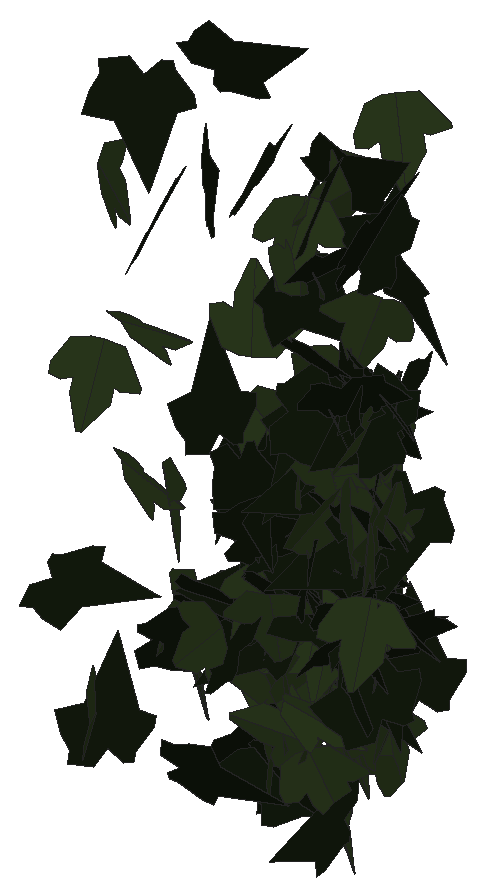
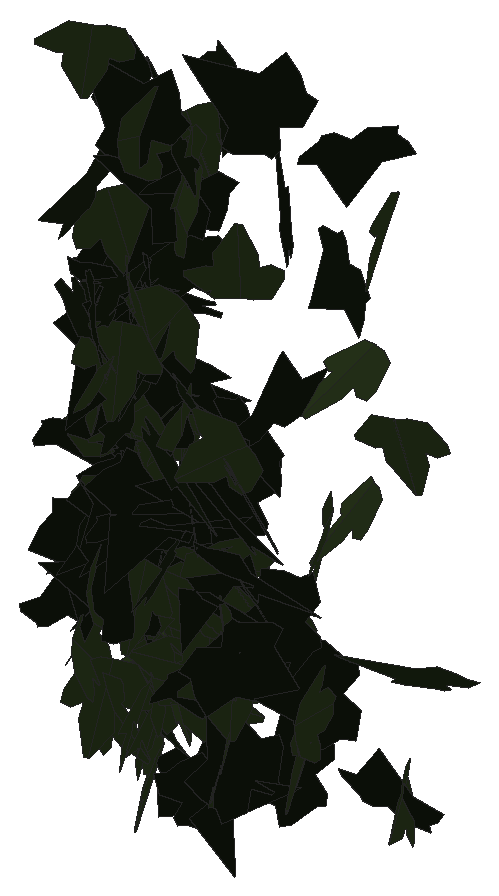
# SketchUp Ruby script. Lengths in inches.
U = 1.inch
M = Sketchup.active_model
def pt(a) = Geom::Point3d.new(a.map { |v| v * U })
def face(e, loops, mat)
  f = e.add_face(loops[0].map { |a| pt(a) })
  loops[1..].each { |l| e.add_face(l.map { |a| pt(a) }).erase! }
  f.material = f.back_material = mat if mat
  f
end
# faces: each face lists its corners as indices into pts; further lists are holes
def faces(e, pts, list, mat = nil) = list.each { |f| face(e, (f[0].is_a?(Array) ? f : [f]).map { |l| l.map { |i| pts[i] } }, mat) }
# xy, xz, yz: faces in a plane at the given z, y or x. An outline is a flat list of corners, or four numbers for a rectangle; further outlines are holes
def ring(l) = l.size == 4 ? [[l[0], l[1]], [l[2], l[1]], [l[2], l[3]], [l[0], l[3]]] : l.each_slice(2).to_a
def flat(e, list, mat, &to3) = list.each { |f| face(e, (f[0].is_a?(Array) ? f : [f]).map { |l| ring(l).map { |u, v| to3.(u, v) } }, mat) }
def xy(e, z, list, mat = nil) = flat(e, list, mat) { |x, y| [x, y, z] }
def xz(e, y, list, mat = nil) = flat(e, list, mat) { |x, z| [x, y, z] }
def yz(e, x, list, mat = nil) = flat(e, list, mat) { |y, z| [x, y, z] }
def lines(e, pts, list) = list.each { |a, b| e.add_line(pt(pts[a]), pt(pts[b])) }
# prism: a flat outline (further loops are holes) pulled along v
def prism(e, loops, v, mat = nil)
  f = face(e, loops, mat); d = Geom::Vector3d.new(v.map { |x| x * U })
  f.pushpull(f.normal.samedirection?(d) ? d.length : -d.length)
end
def box(e, o, s, mat = nil) = prism(e, [[o, [o[0] + s[0], o[1], o[2]], [o[0] + s[0], o[1] + s[1], o[2]], [o[0], o[1] + s[1], o[2]]]], [0, 0, s[2]], mat)
def at(x, y, z, deg = 0) = Geom::Transformation.translation(pt([x, y, z])) * Geom::Transformation.rotation(ORIGIN, Z_AXIS, deg.degrees)
def axes(o, x, y, z) = Geom::Transformation.new([*x, 0, *y, 0, *z, 0, *pt(o).to_a, 1])
def part(name) = M.definitions.add(name)
# library, detail: a bought-in or finely detailed component or shape, given as its bounding box
def library(name, o, s) = part(name).tap { |d| box(d.entities, o, s) }
def detail(e, o, s) = box(e.add_group.entities, o, s)
def put(e, d, t, mat = nil) = e.add_instance(d, t).tap { |i| i.material = mat if mat }
def group(e, t, mat = nil) = e.add_group.tap { |g| g.transformation = t; g.material = mat if mat }.entities
root = M.entities
M.materials.add("efeu1").color = [18, 25, 13]
M.materials.add("efeu2").color = [43, 57, 29]
c1 = part("ivyleaf_10")
p = [[0,0.5,-0.03],[-0.0625,2.02,-0.43],[-0.19,2.01,-0.46],[-0.54,1.05,-0.29],[-0.52,0.625,-0.18],[-0.83,0.76,-0.28],
  [-1.16,0.64,-0.33],[-1.15,0.33,-0.24],[-0.77,-0.39,0.02],[-0.3,-0.51,0.16],[0.04,-0.48,0.23],[-0.02,2.01,-0.4375],
  [-0.06,2.01,-0.43],[0.04,-0.49,0.23],[0.67,-0.49,0.14],[1.38,0.36,-0.2],[1.375,0.51,-0.24],[0.81,0.65,-0.19],
  [0.62,0.59,-0.15],[0.6,1.09,-0.28],[0.5,1.23,-0.31]]
faces(c1.entities,p,[[0,1,2,3,4,5,6,7,8,9,10],[11,12,0,13,14,15,16,17,18,19,20]],"efeu2")
c2 = part("ivyleaf_9")
p = [[1.54,2.16,1.25],[1.36,2.04,1.19],[-0.21,0.99,0.68],[-0.71,1.11,0.82],[-0.85,0.86,0.67],[-0.8,0.17,0.21],
  [-0.9,-0.01,0.1],[-0.67,-0.16,-0.02],[-0.08,-0.08,-0.05],[-0.03,-0.6,-0.4],[0.65,-0.88,-0.66],[0.83,-0.6,-0.49],
  [1.29,-0.42,-0.43],[1.8125,-0.07,-0.26],[1.21,0.44,0.15]]
faces(c2.entities,p,[[0,1,2,3,4,5,6,7,8,9,10,11,12,13,14]],"efeu1")
put(root,c1,axes([48.09,222.28,228.71],[0.48121,0.12764,-0.04631],[-0.04222,-0.02142,-0.49775],[-0.12905,0.48296,-0.00983]))
put(root,c1,axes([51.44,222.29,231.98],[0.3346,0.34907,-0.12725],[-0.09542,-0.08477,-0.48344],[-0.35908,0.3478,0.00989]))
put(root,c1,axes([52.53,222.28,226.43],[0.43327,0.24382,-0.05315],[-0.05124,-0.0173,-0.49707],[-0.24423,0.43618,0.01]))
put(root,c1,axes([52.73,222.16,227.76],[-0.277,0.39289,0.13752],[-0.21085,0.01,-0.45326],[-0.35891,-0.30909,0.16014]))
put(root,c2,axes([50.6,222.04,225.375],[-0.24115,0.33133,0.28647],[-0.16642,0.23319,-0.40979],[-0.40515,-0.293,-0.00219]))
put(root,c2,axes([50.43,222.33,227.94],[-0.20338,-0.06794,-0.45168],[0.42569,0.15107,-0.2144],[0.1656,-0.47177,-0.0036]))
put(root,c2,axes([52.35,222.05,229.83],[0.27412,0.39775,-0.12905],[-0.07958,-0.10187,-0.483],[-0.41052,0.28534,0.00746]))
put(root,c1,axes([51.73,222.08,227.43],[0.06277,-0.40407,0.28773],[0.05223,0.2938,0.40119],[-0.49329,-0.02031,0.07909]))
put(root,c2,axes([51.53,222.04,229.23],[0.43302,-0.15738,-0.19423],[0.16184,0.47257,-0.0221],[0.19053,-0.04373,0.4602]))
put(root,c1,axes([50,222.21,225.33],[0.34063,-0.17868,-0.31944],[-0.27529,0.16253,-0.38445],[0.24123,0.43779,0.01234]))
put(root,c2,axes([49.62,222.17,223.22],[0.36236,-0.05395,0.34027],[0.33785,-0.04109,-0.36629],[0.06749,0.49538,0.00668]))
put(root,c2,axes([50.99,221.89,232.46],[-0.00496,0.35477,0.35229],[-0.05096,0.35012,-0.3533],[-0.49737,-0.03941,0.03268]))
put(root,c2,axes([52.56,221.92,231.89],[-0.09163,0.45658,-0.18205],[-0.12965,0.15618,0.45695],[0.47412,0.13095,0.08977]))
put(root,c2,axes([52.13,222.26,223.29],[-0.42088,0.26181,0.06571],[-0.06124,0.02593,-0.49556],[-0.26289,-0.42519,0.01024]))
put(root,c1,axes([48.46,222.05,231.64],[-0.21111,0.38336,0.2418],[-0.12345,0.20802,-0.43759],[-0.43611,-0.24446,0.00682]))
put(root,c2,axes([48.4,222.125,223.1875],[-0.47956,0.0792,0.11727],[0.11495,-0.02368,0.48603],[0.08254,0.49312,0.0045]))
put(root,c1,axes([48.83,222.08,227.37],[0.37792,-0.31183,-0.09967],[0.22466,0.35776,-0.26746],[0.23812,0.15737,0.41053]))
put(root,c2,axes([47.5,222.2,225.28],[0.36048,-0.33587,-0.08514],[0.29595,0.36235,-0.17641],[0.1802,0.07679,0.46004]))
put(root,c1,axes([51.51,222.17,224.71],[0.29066,-0.40681,0.00494],[0.38529,0.2733,-0.16387],[0.13063,0.09907,0.47236]))
put(root,c1,axes([52.25,222.37,228.06],[-0.09953,0.46922,-0.14118],[0.01606,-0.14086,-0.47948],[-0.48973,-0.09998,0.01297]))
put(root,c1,axes([51,222.3,226.04],[-0.44334,-0.23081,-0.01328],[0.01364,0.00255,-0.49981],[0.23079,-0.44353,0.00403]))
put(root,c2,axes([51.51,222.12,230.17],[0.47687,0.09612,-0.11555],[-0.12921,0.06577,-0.47852],[-0.07679,0.48625,0.08757]))
put(root,c1,axes([51.91,222.36,228.42],[-0.45824,-0.1881,-0.06807],[0.0791,-0.01412,-0.4935],[0.18373,-0.46306,0.0427]))
put(root,c2,axes([51.87,222.74,228.13],[-0.01978,-0.18128,-0.46556],[-0.06891,-0.46048,0.18223],[-0.49483,0.07137,-0.00677]))
put(root,c1,axes([51.46,222.1875,231.17],[-0.05036,0.45266,-0.2063],[-0.02036,0.20531,0.45545],[0.49704,0.05428,-0.00225]))
put(root,c1,axes([50.64,222.3,229.93],[0.42439,0.26344,-0.02228],[0.01605,0.01638,0.49947],[0.26389,-0.42465,0.00544]))
put(root,c2,axes([52.6875,222.37,225.01],[-0.45741,-0.19549,0.05063],[0.04972,0.01249,0.49737],[-0.19572,0.46003,0.00801]))
put(root,c2,axes([51.16,222.6,226.31],[-0.04639,0.19704,0.45719],[0.09368,-0.44751,0.20237],[0.48895,0.10444,0.00461]))
put(root,c2,axes([51.43,222.23,231.04],[0.04042,-0.20592,-0.45383],[-0.06745,0.44887,-0.20967],[0.49378,0.07817,0.00851]))
put(root,c2,axes([52.27,222.87,229.03],[-0.18693,-0.30126,0.35257],[-0.11643,-0.33747,-0.35008],[0.44889,-0.21298,0.05602]))
put(root,c1,axes([48.1,222.125,223.48],[0.02576,-0.11307,-0.48637],[-0.11085,0.47357,-0.11596],[0.48688,0.1138,-0.00067]))
put(root,c1,axes([52.41,222.81,228.96],[0.00413,0.14841,-0.47745],[-0.12491,-0.46202,-0.1447],[-0.48413,0.12047,0.03326]))
put(root,c1,axes([51.66,222.31,223.89],[0.41757,0.18759,0.20112],[0.09267,0.24829,-0.42399],[-0.25894,0.39136,0.17259]))
put(root,c2,axes([51.56,222.69,228.68],[-0.45452,-0.20479,-0.03835],[0.03525,0.01511,-0.49853],[0.20535,-0.45589,0.0007]))
put(root,c1,axes([49.11,222.5,227.125],[-0.22957,0.42583,-0.12634],[0.0419,-0.12082,-0.48337],[-0.4422,-0.23252,0.01979]))
put(root,c2,axes([52.81,222.5,229.19],[-0.32799,0.12137,0.35734],[-0.34156,0.10588,-0.34947],[-0.16049,-0.47335,0.01346]))
put(root,c2,axes([50.48,222.27,226.87],[0.22341,0.045,0.44504],[0.43742,0.08206,-0.22788],[-0.09354,0.49116,-0.0027]))
put(root,c1,axes([48.76,222.19,229.4375],[0.45445,-0.19943,-0.06089],[0.17582,0.44498,-0.14519],[0.1121,0.11056,0.47456]))
put(root,c2,axes([48.58,222.63,232.85],[-0.17296,-0.42278,-0.20332],[0.07512,0.18894,-0.45679],[0.46308,-0.18856,-0.00184]))
put(root,c2,axes([51.28,222.49,231.56],[-0.0728,0.39409,0.29899],[0.05807,-0.29331,0.40074],[0.49125,0.09308,-0.00306]))
put(root,c2,axes([52.9,222.36,231.9],[-0.24422,0.23522,0.36746],[-0.27114,0.2481,-0.33902],[-0.34182,-0.36486,0.00637]))
put(root,c2,axes([52.0625,222.27,225.96],[-0.02572,0.49678,0.05051],[-0.0109,0.05,-0.49737],[-0.49922,-0.02669,0.00826]))
put(root,c2,axes([52.18,222.69,227.18],[-0.46901,-0.0103,0.173],[-0.17192,-0.0353,-0.46819],[0.02185,-0.49865,0.02957]))
put(root,c2,axes([49.99,222.41,228.28],[-0.21846,-0.31745,0.31859],[0.18107,0.26213,0.38535],[-0.41169,0.28374,0.00043]))
put(root,c2,axes([52.22,222.29,229.32],[0.11383,-0.05902,0.48328],[-0.12598,0.47584,0.08778],[-0.47029,-0.14175,0.09346]))
put(root,c1,axes([51.37,222.62,227.94],[-0.05387,0.45471,-0.20084],[0.02872,-0.19883,-0.45787],[-0.49626,-0.06087,-0.0047]))
put(root,c1,axes([50.71,222.63,226.11],[0.39975,0.2084,-0.21626],[-0.20328,-0.07728,-0.45023],[-0.22108,0.44788,0.02294]))
put(root,c2,axes([51.95,222.39,227.76],[0.38352,0.20518,-0.2466],[-0.22821,-0.09562,-0.43449],[-0.22545,0.44582,0.0203]))
put(root,c2,axes([52.0625,222.4375,225.89],[0.29918,0.12418,-0.38088],[-0.36429,-0.11346,-0.32314],[-0.16669,0.47086,0.02258]))
put(root,c2,axes([51.46,222.25,230.98],[0.04497,0.4596,-0.19169],[0.0122,0.1914,0.46176],[0.49782,-0.04621,0.006]))
put(root,c1,axes([51.11,222.64,223.99],[0.03124,0.02838,0.49822],[-0.47397,-0.1545,0.03852],[0.15613,-0.47468,0.01726]))
put(root,c1,axes([51.41,222.7,224.24],[0.2328,-0.43837,0.0603],[0.03077,-0.05193,-0.49634],[0.44143,0.2348,0.0028]))
put(root,c2,axes([50.71,222.64,225.95],[-0.36317,0.12513,0.32008],[-0.31605,0.06131,-0.38256],[-0.13499,-0.48019,0.03457]))
put(root,c2,axes([50.73,222.77,225.51],[-0.49759,0.00548,0.04869],[-0.04896,-0.03724,-0.4962],[-0.00181,-0.49858,0.0376]))
put(root,c1,axes([52.49,222.7,227.34],[-0.047,-0.49677,-0.03181],[0.01952,-0.03376,0.49848],[-0.4974,0.04562,0.02257]))
put(root,c2,axes([49.52,222.5,225.57],[0.44997,-0.04403,0.21351],[0.21268,-0.01882,-0.45212],[0.04785,0.4977,0.00179]))
put(root,c2,axes([50.88,222.47,226.23],[0.40205,0.23442,-0.18277],[-0.1743,-0.06312,-0.46437],[-0.24078,0.43711,0.03097]))
put(root,c1,axes([51.03,222.89,230.9375],[-0.10224,-0.08584,0.48185],[0.44581,-0.21949,0.05549],[0.202,0.44097,0.12141]))
put(root,c2,axes([52.17,222.41,226.43],[0.29402,0.40385,-0.02139],[-0.01403,-0.01625,-0.49954],[-0.40417,0.29435,0.00178]))
put(root,c1,axes([50.58,222.7,224.53],[-0.45213,0.06828,-0.20228],[-0.198,0.04307,0.4571],[0.07985,0.49344,-0.01191]))
put(root,c1,axes([52.31,222.78,230.66],[-0.36566,-0.30066,0.16093],[-0.08805,-0.14471,-0.47043],[0.32945,-0.37237,0.05288]))
put(root,c2,axes([52.15,222.5625,226.52],[0.22814,0.23446,-0.37812],[-0.35306,-0.16318,-0.3142],[-0.27074,0.41036,0.0911]))
put(root,c2,axes([51.53,222.81,226.08],[-0.33761,-0.32349,-0.17714],[-0.12845,-0.12198,0.46757],[-0.34572,0.36122,-0.00074]))
put(root,c2,axes([52.2,222.57,225.35],[0.34726,-0.23485,-0.27251],[-0.17664,0.21864,-0.41352],[0.31339,0.38346,0.06888]))
put(root,c2,axes([49.37,222.95,231.32],[-0.0104,0.09201,0.49135],[0.10171,-0.48079,0.09218],[0.48943,0.10187,-0.00872]))
put(root,c2,axes([52.09,222.95,229.58],[0.17314,-0.33921,0.32397],[0.22137,-0.24537,-0.37522],[0.41354,0.27337,0.06522]))
put(root,c2,axes([51.69,222.57,229.26],[0.38175,-0.11537,-0.30159],[-0.28345,0.10395,-0.39856],[0.15466,0.47527,0.01397]))
put(root,c2,axes([48.89,222.35,230.84],[-0.22185,0.25057,-0.37149],[-0.27378,0.25236,0.33371],[0.35473,0.35147,0.02523]))
put(root,c2,axes([51.12,222.48,227.99],[-0.16159,0.33224,0.33691],[-0.19045,0.28024,-0.36769],[-0.43315,-0.24716,0.03598]))
put(root,c1,axes([51.32,222.84,225.57],[0.33872,0.10986,-0.351],[-0.3454,-0.06891,-0.35489],[-0.12636,0.48289,0.02921]))
put(root,c1,axes([51.78,222.83,227.4],[0.46853,-0.17218,-0.02893],[-0.02574,0.01382,-0.49915],[0.17268,0.46922,0.00409]))
put(root,c2,axes([50.74,222.62,226.83],[-0.22959,0.2497,0.36734],[-0.28158,0.23797,-0.33776],[-0.34351,-0.36196,0.03135]))
put(root,c2,axes([48.93,222.49,224.75],[0.1533,0.30837,-0.3625],[0.13277,0.33801,0.34368],[0.45702,-0.20164,0.02175]))
put(root,c1,axes([51.59,223.19,232.08],[0.01462,-0.06482,0.49557],[0.02058,-0.49528,-0.06539],[0.49936,0.02231,-0.01181]))
put(root,c1,axes([51.84,222.95,229.74],[0.34943,-0.31306,0.17289],[0.16036,-0.07889,-0.46697],[0.31966,0.3818,0.04527]))
put(root,c1,axes([51.42,222.875,225.625],[0.49994,0.0078,-0.00098],[-0.00098,0.00001,-0.5],[-0.0078,0.49994,0.00002]))
put(root,c1,axes([51.95,222.79,226.59],[0.38817,0.17714,0.26066],[0.24014,0.10156,-0.42664],[-0.20409,0.45641,-0.00624]))
put(root,c1,axes([51.41,222.79,225.88],[-0.48527,-0.11626,-0.03155],[0.02886,0.01493,-0.49894],[0.11695,-0.48607,-0.00778]))
put(root,c1,axes([50.47,222.89,223.87],[-0.31674,0.3229,-0.21309],[0.14668,-0.1546,-0.45231],[-0.35799,-0.34904,0.00321]))
put(root,c2,axes([52.38,223.08,229.36],[-0.22151,0.04741,-0.44574],[0.41213,-0.17402,-0.22331],[-0.17631,-0.46634,0.03802]))
put(root,c1,axes([51.25,223.2,224.35],[-0.08042,0.10968,-0.48115],[0.04337,-0.48404,-0.11759],[-0.49158,-0.06064,0.06834]))
put(root,c2,axes([52.11,223.09,225.4375],[0.1532,-0.46243,0.11265],[0.0509,-0.10174,-0.48689],[0.47322,0.16065,0.0159]))
put(root,c2,axes([51.79,223.03,228.14],[0.303,-0.34707,0.19424],[0.12134,-0.15188,-0.46066],[0.37877,0.3263,-0.00781]))
put(root,c1,axes([51.3,222.85,229.49],[-0.4154,0.03386,-0.27622],[0.27348,-0.04215,-0.41645],[-0.05149,-0.49707,0.0165]))
put(root,c1,axes([51.86,222.8,224.63],[0.14947,0.00956,0.47704],[-0.47408,0.0595,0.14735],[-0.05395,-0.49636,0.02685]))
put(root,c2,axes([51.97,222.77,226.42],[0.49478,-0.03487,0.06304],[0.06296,-0.00331,-0.49601],[0.03501,0.49877,0.00111]))
put(root,c2,axes([51.6875,223.16,226.59],[-0.25529,-0.42179,-0.08319],[0.05148,0.06607,-0.49293],[0.42682,-0.26025,0.00969]))
put(root,c1,axes([51.52,222.99,225.57],[0.45563,-0.01027,0.20567],[0.20592,0.02668,-0.45485],[-0.00164,0.49918,0.02854]))
put(root,c1,axes([51.89,222.83,227.93],[0.25969,0.11203,0.41233],[0.35556,0.21091,-0.28124],[-0.23694,0.43928,0.02988]))
put(root,c1,axes([50.36,222.93,225.51],[0.32556,-0.35014,-0.14632],[-0.04765,0.15354,-0.47345],[0.37648,0.32222,0.06661]))
put(root,c2,axes([51.86,222.8,226.76],[0.48161,0.12726,-0.04309],[-0.04012,-0.01684,-0.4981],[-0.12823,0.48324,-0.00601]))
put(root,c2,axes([49.96,222.98,223.3],[0.27437,0.3874,0.15698],[-0.08864,-0.12958,0.47471],[0.40849,-0.28832,-0.00243]))
put(root,c1,axes([51.55,222.89,223.05],[-0.28647,0.40805,0.03781],[-0.01599,0.03497,-0.49852],[-0.40948,-0.28683,-0.00698]))
put(root,c2,axes([52.58,222.79,226.01],[0.15325,0.46755,-0.08893],[-0.04076,-0.08019,-0.49184],[-0.47419,0.15799,0.01354]))
put(root,c2,axes([51.5,223.07,232.12],[-0.01733,-0.10886,0.4877],[0.4445,-0.22631,-0.03471],[0.2283,0.43236,0.10462]))
put(root,c2,axes([51.38,223.08,227.76],[-0.42094,0.23689,-0.12921],[0.10909,-0.06959,-0.48297],[-0.2468,-0.43479,0.0069]))
put(root,c1,axes([52.1,223.36,225.53],[0.04751,-0.08988,0.48956],[0.29937,-0.38772,-0.10023],[0.39764,0.30264,0.01698]))
put(root,c2,axes([52.48,223.27,227.74],[-0.29012,-0.4011,-0.07038],[0.04407,0.05498,-0.49501],[0.40483,-0.29343,0.00345]))
put(root,c1,axes([48.69,223.4,224.82],[0.01181,-0.08835,0.49199],[0.23594,-0.43287,-0.0834],[0.44067,0.23413,0.03146]))
put(root,c2,axes([51.15,223.03,226.23],[0.34847,-0.32946,-0.1415],[-0.1043,0.09565,-0.47955],[0.34306,0.36374,-0.00207]))
put(root,c1,axes([50.96,222.78,224.52],[-0.02527,-0.25493,0.42939],[0.07688,0.42282,0.25556],[-0.49341,0.07893,0.01783]))
put(root,c2,axes([50.79,223.01,223.28],[0.18013,0.16343,-0.43686],[-0.38212,-0.21683,-0.23868],[-0.26746,0.41985,0.04678]))
put(root,c2,axes([52.29,223.18,231.14],[0.31128,-0.38752,0.0541],[0.05184,-0.02768,-0.49653],[0.38783,0.31474,0.02294]))
put(root,c2,axes([50.72,223.26,222.91],[-0.18538,-0.01857,0.46399],[-0.46262,-0.03588,-0.18627],[0.04022,-0.49836,-0.00387]))
put(root,c2,axes([52.04,222.82,229.03],[0.36584,0.34034,0.01801],[0.01184,0.01372,-0.49967],[-0.34061,0.36603,0.00198]))
put(root,c2,axes([49.8125,223.3,227.72],[-0.38113,0.00993,-0.32348],[0.31917,-0.07123,-0.37823],[-0.0536,-0.4948,0.04796]))
put(root,c1,axes([50.1,223.1,224.8],[0.32537,0.37915,0.01941],[0.01356,0.01394,-0.49962],[-0.37941,0.32565,-0.00121]))
put(root,c2,axes([52.63,223.09,229.4],[-0.3713,0.33277,-0.03742],[0.02531,-0.02783,-0.49858],[-0.33391,-0.37214,0.00382]))
put(root,c1,axes([51.42,223.08,223.85],[-0.17997,0.4662,-0.01645],[0.00267,-0.01661,-0.49972],[-0.46648,-0.17995,0.00349]))
put(root,c2,axes([51.55,222.84,226.91],[0.28921,0.40535,0.04521],[0.00863,0.04933,-0.49749],[-0.40778,0.28854,0.02154]))
put(root,c2,axes([49.39,223.16,233.07],[0.07623,-0.09813,0.48431],[0.4805,-0.09967,-0.09583],[0.11535,0.48004,0.07911]))
put(root,c1,axes([51.59,223.15,225.75],[-0.49567,0.06349,0.0166],[-0.01681,-0.0006,-0.49972],[-0.06344,-0.49595,0.00273]))
put(root,c1,axes([52.17,223.51,224.71],[0.15129,-0.34328,0.33057],[0.13264,-0.30279,-0.37513],[0.45773,0.2012,-0.00055]))
put(root,c1,axes([51.91,223.18,229.05],[-0.49255,-0.07475,0.0425],[-0.04211,-0.00576,-0.49819],[0.07497,-0.49435,-0.00062]))
put(root,c2,axes([51.49,223.06,225.42],[0.17122,-0.03937,0.46812],[0.46767,0.06134,-0.1659],[-0.04436,0.49466,0.05783]))
put(root,c1,axes([50.44,222.88,223.41],[0.05308,-0.02491,-0.49655],[-0.1385,0.47886,-0.03883],[0.47749,0.14167,0.04394]))
put(root,c2,axes([49.95,223.46,225.43],[-0.00905,0.11538,-0.48642],[-0.07584,-0.48119,-0.11272],[-0.49413,0.07174,0.02621]))
put(root,c1,axes([48.91,223.17,224.32],[-0.31515,0.38813,-0.00616],[0.00833,-0.00118,-0.49993],[-0.38809,-0.31521,-0.00573]))
put(root,c1,axes([51.57,223.12,224.03],[-0.22018,0.44005,0.08877],[-0.02972,0.08437,-0.49193],[-0.44793,-0.2219,-0.011]))
put(root,c1,axes([52.07,223.21,228.59],[-0.11294,0.48647,-0.02428],[0.01159,-0.02223,-0.49937],[-0.48694,-0.11336,-0.00625]))
put(root,c1,axes([50.03,223.18,228.15],[0.2786,0.06945,0.40934],[0.37002,0.18207,-0.28273],[-0.18833,0.46046,0.05005]))
put(root,c1,axes([52.1,223.22,223.83],[-0.17715,0.05965,0.46374],[-0.46691,0.00365,-0.17883],[-0.02472,-0.49642,0.05441]))
put(root,c1,axes([52.24,223.27,233.35],[0.38254,0.31348,0.07345],[0.06141,0.04093,-0.49452],[-0.31605,0.38737,-0.00719]))
put(root,c1,axes([52.03,223.21,224.18],[-0.30075,-0.37503,-0.13749],[0.08399,0.10888,-0.48072],[0.3905,-0.31225,-0.00249]))
put(root,c2,axes([52.66,223.2,224.93],[-0.36977,-0.23841,0.23756],[0.19719,0.13254,0.43994],[-0.27274,0.41904,-0.004]))
put(root,c2,axes([50.36,223.5,225.03],[-0.09589,-0.48487,-0.07552],[0.01189,0.07463,-0.49426],[0.49057,-0.09659,-0.00278]))
